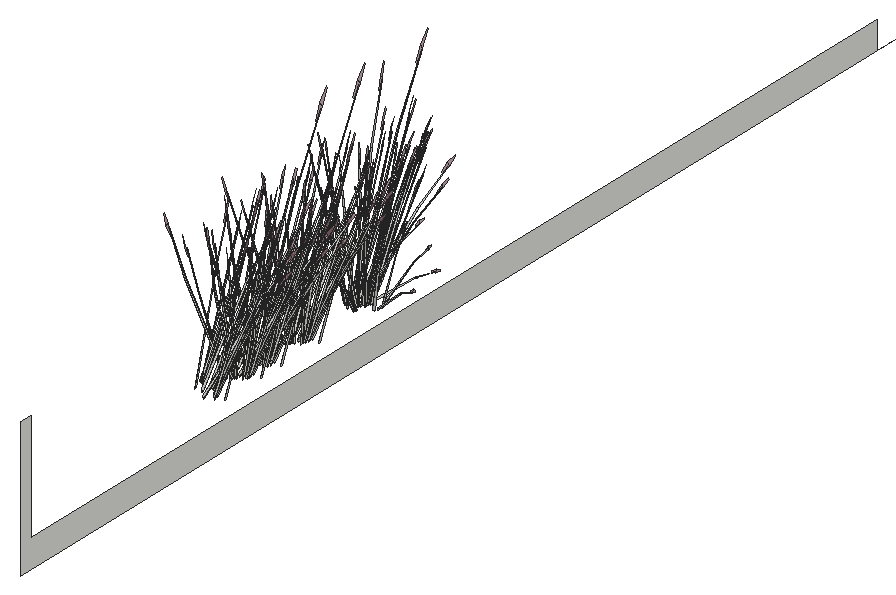
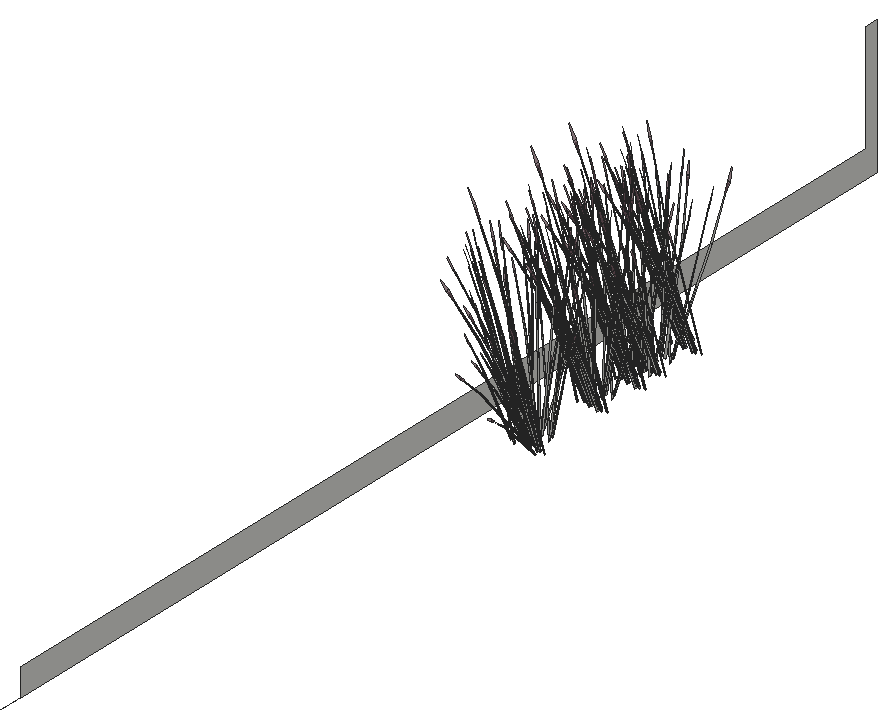
# SketchUp Ruby script. Lengths in inches.
U = 1.inch
M = Sketchup.active_model
def pt(a) = Geom::Point3d.new(a.map { |v| v * U })
def face(e, loops, mat)
  f = e.add_face(loops[0].map { |a| pt(a) })
  loops[1..].each { |l| e.add_face(l.map { |a| pt(a) }).erase! }
  f.material = f.back_material = mat if mat
  f
end
# faces: each face lists its corners as indices into pts; further lists are holes
def faces(e, pts, list, mat = nil) = list.each { |f| face(e, (f[0].is_a?(Array) ? f : [f]).map { |l| l.map { |i| pts[i] } }, mat) }
# xy, xz, yz: faces in a plane at the given z, y or x. An outline is a flat list of corners, or four numbers for a rectangle; further outlines are holes
def ring(l) = l.size == 4 ? [[l[0], l[1]], [l[2], l[1]], [l[2], l[3]], [l[0], l[3]]] : l.each_slice(2).to_a
def flat(e, list, mat, &to3) = list.each { |f| face(e, (f[0].is_a?(Array) ? f : [f]).map { |l| ring(l).map { |u, v| to3.(u, v) } }, mat) }
def xy(e, z, list, mat = nil) = flat(e, list, mat) { |x, y| [x, y, z] }
def xz(e, y, list, mat = nil) = flat(e, list, mat) { |x, z| [x, y, z] }
def yz(e, x, list, mat = nil) = flat(e, list, mat) { |y, z| [x, y, z] }
def lines(e, pts, list) = list.each { |a, b| e.add_line(pt(pts[a]), pt(pts[b])) }
# prism: a flat outline (further loops are holes) pulled along v
def prism(e, loops, v, mat = nil)
  f = face(e, loops, mat); d = Geom::Vector3d.new(v.map { |x| x * U })
  f.pushpull(f.normal.samedirection?(d) ? d.length : -d.length)
end
def box(e, o, s, mat = nil) = prism(e, [[o, [o[0] + s[0], o[1], o[2]], [o[0] + s[0], o[1] + s[1], o[2]], [o[0], o[1] + s[1], o[2]]]], [0, 0, s[2]], mat)
def at(x, y, z, deg = 0) = Geom::Transformation.translation(pt([x, y, z])) * Geom::Transformation.rotation(ORIGIN, Z_AXIS, deg.degrees)
def axes(o, x, y, z) = Geom::Transformation.new([*x, 0, *y, 0, *z, 0, *pt(o).to_a, 1])
def part(name) = M.definitions.add(name)
# library, detail: a bought-in or finely detailed component or shape, given as its bounding box
def library(name, o, s) = part(name).tap { |d| box(d.entities, o, s) }
def detail(e, o, s) = box(e.add_group.entities, o, s)
def put(e, d, t, mat = nil) = e.add_instance(d, t).tap { |i| i.material = mat if mat }
def group(e, t, mat = nil) = e.add_group.tap { |g| g.transformation = t; g.material = mat if mat }.entities
root = M.entities
M.materials.add("LightPink_Translucent").color = [144, 107, 117]
M.materials["LightPink_Translucent"].alpha = 0.75
c1 = part("blade")
p = [[2.15,0.21,22],[0,0.17,0],[0.09,0.45,0],[2.18,0.31,22],[2.29,0.31,22],[0.38,0.45,0],
  [2.48,0.24,33],[2.49,0.24,33],[2.48,0.22,33]]
faces(c1.entities,p,[[0,1,2,3],[4,5,2,3],[6,3,4,7],[8,0,3,6]])
c2 = part("seeds")
p = [[0.3,-0.1,1.38],[-0.01,-0.03,1.59],[-0.01,-0.03,0.03],[0.14,-0.07,-0.07],[0.29,-0.03,3],[0.15,0.01,3.11]]
faces(c2.entities,p,[[0,1,2,3],[1,0,4,5]],"LightPink_Translucent")
c3 = part("blade with seeds")
put(c3.entities,c1,at(0,0,0))
put(c3.entities,c2,axes([2.4,0.25,30.99],[1.5799,-0.05474,1.17369],[-0.12525,1.92788,0.29478],[-0.07173,-0.02425,1.56792]))
yz(root,288,[[291,126,291,156,294,156,294,132,525,132,525,126]])
p = [[288,525,126],[288,531,126]]
lines(root,p,[[0,1]])
put(root,c3,axes([271,359.68,126.52],[-0.0219,-0.25042,1.71376],[0.94901,0.16613,0.13857],[-0.0587,0.35688,0.73262]))
put(root,c3,axes([271,369.5,126.55],[-0.0219,-0.25042,1.71376],[0.94901,0.16613,0.13857],[-0.0587,0.35688,0.73262]))
put(root,c3,axes([271,375.11,126.42],[-0.0219,-0.25042,1.71376],[0.94901,0.16613,0.13857],[-0.0587,0.35688,0.73262]))
put(root,c3,axes([271,385.48,126.46],[-0.0219,-0.25042,1.71376],[0.94901,0.16613,0.13857],[-0.0587,0.35688,0.73262]))
put(root,c3,axes([271,402.59,125.79],[-0.0219,-0.25042,1.71376],[0.94901,0.16613,0.13857],[-0.0587,0.35688,0.73262]))
put(root,c3,axes([272.94,365.45,127.66],[-0.42698,-0.53052,-0.71045],[0.87893,-0.29566,0.08574],[-0.09984,-0.25633,1.00501]))
put(root,c3,axes([272.94,381.43,127.5625],[-0.42698,-0.53052,-0.71045],[0.87893,-0.29566,0.08574],[-0.09984,-0.25633,1.00501]))
put(root,c3,axes([273.11,398.62,126.97],[-0.2697,0.50175,0.35414],[-0.78684,-0.14635,-0.4572],[-0.07215,-0.20201,0.87481]))
put(root,c3,axes([271.67,403.87,126.98],[-0.88151,-0.17057,0.53283],[0.30143,-0.56078,0.43934],[0.05297,0.22053,1.10256]))
put(root,c3,axes([271.4375,403.91,126.64],[-0.6592,0.22175,0.0643],[-0.32265,-0.40436,0.50621],[0.06366,0.17825,0.77189]))
put(root,c3,axes([273.02,365,127.2],[0.2697,-0.50175,-0.35414],[0.78684,0.14635,0.4572],[-0.07215,-0.20201,0.87481]))
put(root,c3,axes([273.02,370.61,127.07],[0.2697,-0.50175,-0.35414],[0.78684,0.14635,0.4572],[-0.07215,-0.20201,0.87481]))
put(root,c3,axes([273.02,380.98,127.11],[0.2697,-0.50175,-0.35414],[0.78684,0.14635,0.4572],[-0.07215,-0.20201,0.87481]))
put(root,c3,axes([271.77,361.08,127.17],[-0.2697,0.50175,-0.35414],[-0.78684,-0.14635,0.4572],[0.07215,0.20201,0.87481]))
put(root,c3,axes([271.77,370.9,127.2],[-0.2697,0.50175,-0.35414],[-0.78684,-0.14635,0.4572],[0.07215,0.20201,0.87481]))
put(root,c3,axes([271.77,376.51,127.07],[-0.2697,0.50175,-0.35414],[-0.78684,-0.14635,0.4572],[0.07215,0.20201,0.87481]))
put(root,c3,axes([271.77,386.875,127.11],[-0.2697,0.50175,-0.35414],[-0.78684,-0.14635,0.4572],[0.07215,0.20201,0.87481]))
put(root,c3,axes([273.35,398.16,126.64],[0.6592,-0.22175,0.0643],[0.32265,0.40436,0.50621],[-0.06366,-0.17825,0.77189]))
put(root,c3,axes([271.21,404.875,126.63],[0.1134,0.10507,1.74944],[0.91515,0.04128,-0.27667],[0.09203,0.23172,0.14031]))
put(root,c3,axes([273.12,398.2,126.65],[0.88151,0.17057,0.48003],[-0.30143,0.56078,0.3958],[-0.05297,-0.22053,0.9933]))
put(root,c3,axes([271.68,403.46,126.97],[0.2697,-0.50175,0.35414],[0.78684,0.14635,-0.4572],[0.07215,0.20201,0.87481]))
put(root,c3,axes([271.85,360.625,127.625],[0.42698,0.53052,-0.71045],[-0.87893,0.29566,0.08574],[0.09984,0.25633,1.00501]))
put(root,c3,axes([271.85,370.45,127.66],[0.42698,0.53052,-0.71045],[-0.87893,0.29566,0.08574],[0.09984,0.25633,1.00501]))
put(root,c3,axes([271.85,386.42,127.5625],[0.42698,0.53052,-0.71045],[-0.87893,0.29566,0.08574],[0.09984,0.25633,1.00501]))
put(root,c3,axes([272.17,360.73,127.33],[0.87941,0.16356,-0.51099],[-0.30143,0.56078,-0.3958],[0.08064,0.22578,0.97773]))
put(root,c3,axes([272.17,370.55,127.36],[0.87941,0.16356,-0.51099],[-0.30143,0.56078,-0.3958],[0.08064,0.22578,0.97773]))
put(root,c3,axes([272.17,376.17,127.23],[0.87941,0.16356,-0.51099],[-0.30143,0.56078,-0.3958],[0.08064,0.22578,0.97773]))
put(root,c3,axes([272.17,386.53,127.26],[0.87941,0.16356,-0.51099],[-0.30143,0.56078,-0.3958],[0.08064,0.22578,0.97773]))
put(root,c3,axes([271.42,360.76,127.68],[0.87543,-0.30377,-0.1216],[0.4302,0.53915,-0.67495],[0.1155,0.2272,1.02557]))
put(root,c3,axes([271.42,376.19,127.58],[0.87543,-0.30377,-0.1216],[0.4302,0.53915,-0.67495],[0.1155,0.2272,1.02557]))
put(root,c3,axes([271.42,386.56,127.61],[0.87543,-0.30377,-0.1216],[0.4302,0.53915,-0.67495],[0.1155,0.2272,1.02557]))
put(root,c3,axes([271.42,403.67,126.95],[0.87543,-0.30377,-0.1216],[0.4302,0.53915,-0.67495],[0.1155,0.2272,1.02557]))
put(root,c3,axes([275.89,397.65,126.625],[-0.09085,0.04984,1.77383],[-0.89014,-0.16814,-0.16761],[-0.03222,-0.21748,0.31391]))
put(root,c3,axes([275.19,371.61,127.58],[-0.98321,-0.03233,-0.1216],[0.02687,-0.61208,-0.67495],[0.0683,-0.23574,1.02557]))
put(root,c3,axes([275.19,381.98,127.61],[-0.98321,-0.03233,-0.1216],[0.02687,-0.61208,-0.67495],[0.0683,-0.23574,1.02557]))
put(root,c3,axes([275.19,399.09,126.95],[-0.98321,-0.03233,-0.1216],[0.02687,-0.61208,-0.67495],[0.0683,-0.23574,1.02557]))
put(root,c3,axes([274.81,399.18,126.97],[-0.60531,0.34352,0.35414],[-0.573,-0.39225,-0.4572],[0.08718,-0.19929,0.87481]))
put(root,c3,axes([274.52,365.77,127.36],[-0.64041,-0.4384,-0.51099],[0.67652,-0.38394,-0.3958],[0.09744,-0.22274,0.97773]))
put(root,c3,axes([274.52,371.38,127.23],[-0.64041,-0.4384,-0.51099],[0.67652,-0.38394,-0.3958],[0.09744,-0.22274,0.97773]))
put(root,c3,axes([274.52,381.74,127.26],[-0.64041,-0.4384,-0.51099],[0.67652,-0.38394,-0.3958],[0.09744,-0.22274,0.97773]))
put(root,c3,axes([273.87,403.73,126.65],[-0.88979,0.14973,0.48003],[-0.15442,-0.58737,0.3958],[0.20926,0.17311,0.9933]))
put(root,c3,axes([273.7,403.85,126.64],[-0.4066,0.41448,0.0643],[-0.57901,-0.24131,0.50621],[0.18719,0.13288,0.77189]))
put(root,c3,axes([272.67,359.57,126.52],[-0.2045,-0.20949,1.71376],[0.94495,-0.17636,0.13857],[0.21357,0.32887,0.73262]))
put(root,c3,axes([272.67,369.4,126.55],[-0.2045,-0.20949,1.71376],[0.94495,-0.17636,0.13857],[0.21357,0.32887,0.73262]))
put(root,c3,axes([272.67,375.01,126.42],[-0.2045,-0.20949,1.71376],[0.94495,-0.17636,0.13857],[0.21357,0.32887,0.73262]))
put(root,c3,axes([272.67,385.37,126.46],[-0.2045,-0.20949,1.71376],[0.94495,-0.17636,0.13857],[0.21357,0.32887,0.73262]))
put(root,c3,axes([272.67,402.48,125.79],[-0.2045,-0.20949,1.71376],[0.94495,-0.17636,0.13857],[0.21357,0.32887,0.73262]))
put(root,c3,axes([274.72,365.97,127.66],[0.02328,-0.60353,-0.71045],[0.98022,0.04053,0.08574],[0.10344,-0.25568,1.00501]))
put(root,c3,axes([274.72,381.95,127.5625],[0.02328,-0.60353,-0.71045],[0.98022,0.04053,0.08574],[0.10344,-0.25568,1.00501]))
put(root,c3,axes([273.57,403.375,126.97],[-0.13817,-0.52554,0.35414],[0.78985,-0.13877,-0.4572],[0.21215,0.1506,0.87481]))
put(root,c3,axes([274.1,372.875,127.02],[-0.77304,-0.33901,1.38283],[0.81626,-0.52782,0.59665],[0.24941,0.31809,1.33663]))
put(root,c3,axes([274.1,383.24,127.05],[-0.77304,-0.33901,1.38283],[0.81626,-0.52782,0.59665],[0.24941,0.31809,1.33663]))
put(root,c3,axes([274.1,400.35,126.39],[-0.77304,-0.33901,1.38283],[0.81626,-0.52782,0.59665],[0.24941,0.31809,1.33663]))
put(root,c3,axes([275.12,365.61,127.2],[0.60531,-0.34352,-0.35414],[0.573,0.39225,0.4572],[0.08718,-0.19929,0.87481]))
put(root,c3,axes([275.12,371.22,127.07],[0.60531,-0.34352,-0.35414],[0.573,0.39225,0.4572],[0.08718,-0.19929,0.87481]))
put(root,c3,axes([275.12,381.58,127.11],[0.60531,-0.34352,-0.35414],[0.573,0.39225,0.4572],[0.08718,-0.19929,0.87481]))
put(root,c3,axes([272.8,404.11,126.625],[0.00265,-0.07899,1.77383],[0.76665,-0.34851,-0.16761],[0.2663,0.12439,0.31391]))
put(root,c3,axes([275.36,398.87,126.64],[0.73517,0.0304,0.0643],[-0.02016,0.45906,0.50621],[0.07693,-0.17585,0.77189]))
put(root,c3,axes([276.09,398.11,126.63],[-0.00864,-0.12985,1.74944],[-0.72937,-0.3753,-0.27667],[0.11277,-0.2275,0.14031]))
put(root,c3,axes([275.12,398.83,126.65],[0.63704,0.44518,0.48003],[-0.67652,0.38394,0.3958],[0.11751,-0.20886,0.9933]))
put(root,c3,axes([275.86,400.24,126.97],[-0.77872,0.09325,0.35414],[-0.20563,-0.53305,-0.4572],[0.22316,-0.14318,0.87481]))
put(root,c3,axes([273.62,365.66,126.55],[-0.16657,0.22426,1.71376],[-0.69879,-0.4641,0.13857],[0.31524,-0.28926,0.73262]))
put(root,c3,axes([273.62,371.28,126.42],[-0.16657,0.22426,1.71376],[-0.69879,-0.4641,0.13857],[0.31524,-0.28926,0.73262]))
put(root,c3,axes([273.62,381.64,126.46],[-0.16657,0.22426,1.71376],[-0.69879,-0.4641,0.13857],[0.31524,-0.28926,0.73262]))
put(root,c3,axes([273.62,398.75,125.79],[-0.16657,0.22426,1.71376],[-0.69879,-0.4641,0.13857],[0.31524,-0.28926,0.73262]))
put(root,c3,axes([273.5,360.74,127.68],[0.53309,-0.55848,-0.1216],[0.77201,0.32175,-0.67495],[0.26836,0.15779,1.02557]))
put(root,c3,axes([273.5,376.17,127.58],[0.53309,-0.55848,-0.1216],[0.77201,0.32175,-0.67495],[0.26836,0.15779,1.02557]))
put(root,c3,axes([273.5,386.53,127.61],[0.53309,-0.55848,-0.1216],[0.77201,0.32175,-0.67495],[0.26836,0.15779,1.02557]))
put(root,c3,axes([273.5,403.65,126.95],[0.53309,-0.55848,-0.1216],[0.77201,0.32175,-0.67495],[0.26836,0.15779,1.02557]))
put(root,c3,axes([276.26,372.82,127.58],[-0.82753,-0.35977,-0.1216],[0.47675,-0.52101,-0.67495],[0.2338,-0.18111,1.02557]))
put(root,c3,axes([276.26,383.18,127.61],[-0.82753,-0.35977,-0.1216],[0.47675,-0.52101,-0.67495],[0.2338,-0.18111,1.02557]))
put(root,c3,axes([276.26,400.29,126.95],[-0.82753,-0.35977,-0.1216],[0.47675,-0.52101,-0.67495],[0.2338,-0.18111,1.02557]))
put(root,c3,axes([274.13,360.46,127.33],[0.88277,-0.1551,-0.51099],[0.15442,0.58737,-0.3958],[0.23711,0.16832,0.97773]))
put(root,c3,axes([274.13,370.28,127.36],[0.88277,-0.1551,-0.51099],[0.15442,0.58737,-0.3958],[0.23711,0.16832,0.97773]))
put(root,c3,axes([274.13,375.89,127.23],[0.88277,-0.1551,-0.51099],[0.15442,0.58737,-0.3958],[0.23711,0.16832,0.97773]))
put(root,c3,axes([274.13,386.26,127.26],[0.88277,-0.1551,-0.51099],[0.15442,0.58737,-0.3958],[0.23711,0.16832,0.97773]))
put(root,c3,axes([275.14,402.66,126.97],[-0.50902,-0.40851,0.35414],[0.58122,-0.38671,-0.4572],[0.29531,0.05884,0.87481]))
put(root,c3,axes([275.61,403.03,126.64],[-0.04505,0.49615,0.0643],[-0.68022,-0.0136,0.50621],[0.26056,0.05192,0.77189]))
put(root,c3,axes([275.67,402.875,126.65],[-0.65964,0.42992,0.48003],[-0.5689,-0.45657,0.3958],[0.30948,0.0793,0.9933]))
put(root,c3,axes([275.85,366.78,127.36],[-0.22982,-0.59576,-0.51099],[0.87033,-0.10422,-0.3958],[0.24941,-0.16002,0.97773]))
put(root,c3,axes([275.85,372.39,127.23],[-0.22982,-0.59576,-0.51099],[0.87033,-0.10422,-0.3958],[0.24941,-0.16002,0.97773]))
put(root,c3,axes([275.85,382.75,127.26],[-0.22982,-0.59576,-0.51099],[0.87033,-0.10422,-0.3958],[0.24941,-0.16002,0.97773]))
put(root,c3,axes([277.38,360.03,126.57],[-0.17122,-0.54847,-0.03492],[0.80929,-0.12609,-0.15832],[0.169,0.03477,0.52218]))
put(root,c3,axes([277.38,369.85,126.6],[-0.17122,-0.54847,-0.03492],[0.80929,-0.12609,-0.15832],[0.169,0.03477,0.52218]))
put(root,c3,axes([277.38,375.47,126.48],[-0.17122,-0.54847,-0.03492],[0.80929,-0.12609,-0.15832],[0.169,0.03477,0.52218]))
put(root,c3,axes([277.38,385.83,126.51],[-0.17122,-0.54847,-0.03492],[0.80929,-0.12609,-0.15832],[0.169,0.03477,0.52218]))
put(root,c3,axes([277.38,402.94,125.84],[-0.17122,-0.54847,-0.03492],[0.80929,-0.12609,-0.15832],[0.169,0.03477,0.52218]))
put(root,c3,axes([275.98,401.52,126.97],[-0.74348,-0.18202,0.35414],[0.21685,-0.53102,-0.4572],[0.29933,-0.04869,0.87481]))
put(root,c3,axes([276.5625,400.16,126.64],[0.61415,0.2744,0.0643],[-0.35756,0.39076,0.50621],[0.1969,-0.12633,0.77189]))
put(root,c3,axes([276.39,400.04,126.65],[0.22187,0.60049,0.48003],[-0.87033,0.10422,0.3958],[0.25651,-0.14123,0.9933]))
put(root,c3,axes([274.04,358.92,126.52],[-0.3323,-0.11241,1.71376],[0.68769,-0.4716,0.13857],[0.42861,0.21275,0.73262]))
put(root,c3,axes([274.04,368.74,126.55],[-0.3323,-0.11241,1.71376],[0.68769,-0.4716,0.13857],[0.42861,0.21275,0.73262]))
put(root,c3,axes([274.04,374.36,126.42],[-0.3323,-0.11241,1.71376],[0.68769,-0.4716,0.13857],[0.42861,0.21275,0.73262]))
put(root,c3,axes([274.04,384.72,126.46],[-0.3323,-0.11241,1.71376],[0.68769,-0.4716,0.13857],[0.42861,0.21275,0.73262]))
put(root,c3,axes([274.04,401.83,125.79],[-0.3323,-0.11241,1.71376],[0.68769,-0.4716,0.13857],[0.42861,0.21275,0.73262]))
put(root,c3,axes([278.3,400.14,126.625],[-0.11685,-0.00496,1.77383],[-0.48522,-0.53096,-0.16761],[0.19486,-0.17458,0.31391]))
put(root,c3,axes([276.49,366.84,127.2],[0.77872,-0.09325,-0.35414],[0.20563,0.53305,0.4572],[0.22316,-0.14318,0.87481]))
put(root,c3,axes([276.49,372.45,127.07],[0.77872,-0.09325,-0.35414],[0.20563,0.53305,0.4572],[0.22316,-0.14318,0.87481]))
put(root,c3,axes([276.49,382.82,127.11],[0.77872,-0.09325,-0.35414],[0.20563,0.53305,0.4572],[0.22316,-0.14318,0.87481]))
put(root,c3,axes([275.875,367.02,127.66],[0.4673,-0.51481,-0.71045],[0.81887,0.36587,0.08574],[0.27902,-0.18652,1.00501]))
put(root,c3,axes([275.875,382.99,127.5625],[0.4673,-0.51481,-0.71045],[0.81887,0.36587,0.08574],[0.27902,-0.18652,1.00501]))
put(root,c3,axes([276.66,401.68,126.64],[0.32857,0.44488,0.0643],[-0.59916,0.21775,0.50621],[0.26412,-0.04296,0.77189]))
put(root,c3,axes([275.87,359.97,127.17],[0.50902,0.40851,-0.35414],[-0.58122,0.38671,0.4572],[0.29531,0.05884,0.87481]))
put(root,c3,axes([275.87,369.79,127.2],[0.50902,0.40851,-0.35414],[-0.58122,0.38671,0.4572],[0.29531,0.05884,0.87481]))
put(root,c3,axes([275.87,375.4,127.07],[0.50902,0.40851,-0.35414],[-0.58122,0.38671,0.4572],[0.29531,0.05884,0.87481]))
put(root,c3,axes([275.87,385.77,127.11],[0.50902,0.40851,-0.35414],[-0.58122,0.38671,0.4572],[0.29531,0.05884,0.87481]))
put(root,c3,axes([275.28,360.01,127.68],[0.0479,-0.66354,-0.1216],[0.90696,0.01814,-0.67495],[0.3493,0.04609,1.02557]))
put(root,c3,axes([275.28,375.45,127.58],[0.0479,-0.66354,-0.1216],[0.90696,0.01814,-0.67495],[0.3493,0.04609,1.02557]))
put(root,c3,axes([275.28,385.8125,127.61],[0.0479,-0.66354,-0.1216],[0.90696,0.01814,-0.67495],[0.3493,0.04609,1.02557]))
put(root,c3,axes([275.28,402.92,126.95],[0.0479,-0.66354,-0.1216],[0.90696,0.01814,-0.67495],[0.3493,0.04609,1.02557]))
put(root,c3,axes([276.29,358.79,127.68],[-0.45012,-0.59081,-0.1216],[0.79888,-0.29033,-0.67495],[0.33665,-0.07795,1.02557]))
put(root,c3,axes([276.29,374.22,127.58],[-0.45012,-0.59081,-0.1216],[0.79888,-0.29033,-0.67495],[0.33665,-0.07795,1.02557]))
put(root,c3,axes([276.29,384.58,127.61],[-0.45012,-0.59081,-0.1216],[0.79888,-0.29033,-0.67495],[0.33665,-0.07795,1.02557]))
put(root,c3,axes([276.29,401.7,126.95],[-0.45012,-0.59081,-0.1216],[0.79888,-0.29033,-0.67495],[0.33665,-0.07795,1.02557]))
put(root,c3,axes([276.59,401.53,126.65],[-0.25275,0.59491,0.48003],[-0.83094,-0.20343,0.3958],[0.32677,-0.03575,0.9933]))
put(root,c3,axes([276.07,402.53,126.63],[0.19191,-0.01103,1.74944],[0.52639,-0.5069,-0.27667],[0.34136,0.06691,0.14031]))
put(root,c3,axes([276.26,358.28,127.33],[0.24236,-0.59349,-0.51099],[0.83094,0.20343,-0.3958],[0.33455,-0.05442,0.97773]))
put(root,c3,axes([276.26,368.1,127.36],[0.24236,-0.59349,-0.51099],[0.83094,0.20343,-0.3958],[0.33455,-0.05442,0.97773]))
put(root,c3,axes([276.26,373.71,127.23],[0.24236,-0.59349,-0.51099],[0.83094,0.20343,-0.3958],[0.33455,-0.05442,0.97773]))
put(root,c3,axes([276.26,384.08,127.26],[0.24236,-0.59349,-0.51099],[0.83094,0.20343,-0.3958],[0.33455,-0.05442,0.97773]))
put(root,c3,axes([276.76,358.55,127.17],[0.74348,0.18202,-0.35414],[-0.21685,0.53102,0.4572],[0.29933,-0.04869,0.87481]))
put(root,c3,axes([276.76,368.37,127.2],[0.74348,0.18202,-0.35414],[-0.21685,0.53102,0.4572],[0.29933,-0.04869,0.87481]))
put(root,c3,axes([276.76,373.99,127.07],[0.74348,0.18202,-0.35414],[-0.21685,0.53102,0.4572],[0.29933,-0.04869,0.87481]))
put(root,c3,axes([276.76,384.35,127.11],[0.74348,0.18202,-0.35414],[-0.21685,0.53102,0.4572],[0.29933,-0.04869,0.87481]))
put(root,c3,axes([275.33,359.69,127.625],[0.89428,0.01571,-0.71045],[-0.06006,0.66153,0.08574],[0.37886,0.06981,1.00501]))
put(root,c3,axes([275.33,369.52,127.66],[0.89428,0.01571,-0.71045],[-0.06006,0.66153,0.08574],[0.37886,0.06981,1.00501]))
put(root,c3,axes([275.33,385.49,127.5625],[0.89428,0.01571,-0.71045],[-0.06006,0.66153,0.08574],[0.37886,0.06981,1.00501]))
put(root,c3,axes([278.09,403.45,126.625],[-0.08089,-0.05712,1.77383],[0.17695,-0.61228,-0.16761],[0.31864,-0.03912,0.31391]))
put(root,c3,axes([274.74,357.89,126.52],[-0.37107,0.01478,1.71376],[0.24616,-0.64047,0.13857],[0.5288,0.03961,0.73262]))
put(root,c3,axes([274.74,367.71,126.55],[-0.37107,0.01478,1.71376],[0.24616,-0.64047,0.13857],[0.5288,0.03961,0.73262]))
put(root,c3,axes([274.74,373.33,126.42],[-0.37107,0.01478,1.71376],[0.24616,-0.64047,0.13857],[0.5288,0.03961,0.73262]))
put(root,c3,axes([274.74,383.69,126.46],[-0.37107,0.01478,1.71376],[0.24616,-0.64047,0.13857],[0.5288,0.03961,0.73262]))
put(root,c3,axes([274.74,400.8,125.79],[-0.37107,0.01478,1.71376],[0.24616,-0.64047,0.13857],[0.5288,0.03961,0.73262]))
put(root,c3,axes([276.1,358.5,127.625],[0.78611,-0.28816,-0.71045],[0.4381,0.59317,0.08574],[0.37982,-0.06738,1.00501]))
put(root,c3,axes([276.1,368.32,127.66],[0.78611,-0.28816,-0.71045],[0.4381,0.59317,0.08574],[0.37982,-0.06738,1.00501]))
put(root,c3,axes([276.1,384.29,127.5625],[0.78611,-0.28816,-0.71045],[0.4381,0.59317,0.08574],[0.37982,-0.06738,1.00501]))
put(root,c3,axes([278.74,400.77,126.63],[0.12414,-0.09938,1.74944],[-0.15889,-0.60963,-0.27667],[0.31148,-0.11559,0.14031]))
